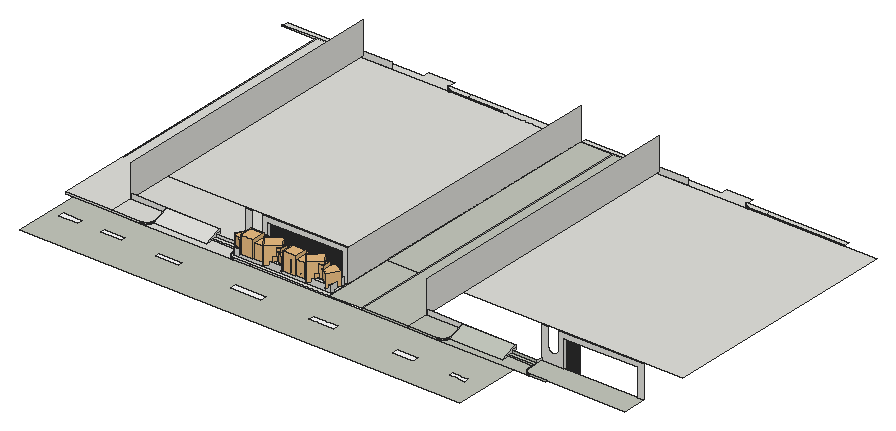
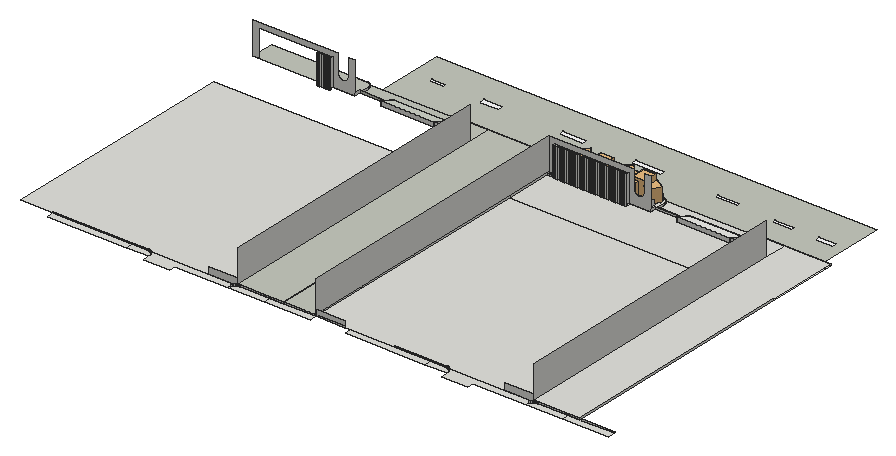
# SketchUp Ruby script. Lengths in inches.
U = 1.inch
M = Sketchup.active_model
def pt(a) = Geom::Point3d.new(a.map { |v| v * U })
def face(e, loops, mat)
  f = e.add_face(loops[0].map { |a| pt(a) })
  loops[1..].each { |l| e.add_face(l.map { |a| pt(a) }).erase! }
  f.material = f.back_material = mat if mat
  f
end
# faces: each face lists its corners as indices into pts; further lists are holes
def faces(e, pts, list, mat = nil) = list.each { |f| face(e, (f[0].is_a?(Array) ? f : [f]).map { |l| l.map { |i| pts[i] } }, mat) }
# xy, xz, yz: faces in a plane at the given z, y or x. An outline is a flat list of corners, or four numbers for a rectangle; further outlines are holes
def ring(l) = l.size == 4 ? [[l[0], l[1]], [l[2], l[1]], [l[2], l[3]], [l[0], l[3]]] : l.each_slice(2).to_a
def flat(e, list, mat, &to3) = list.each { |f| face(e, (f[0].is_a?(Array) ? f : [f]).map { |l| ring(l).map { |u, v| to3.(u, v) } }, mat) }
def xy(e, z, list, mat = nil) = flat(e, list, mat) { |x, y| [x, y, z] }
def xz(e, y, list, mat = nil) = flat(e, list, mat) { |x, z| [x, y, z] }
def yz(e, x, list, mat = nil) = flat(e, list, mat) { |y, z| [x, y, z] }
def lines(e, pts, list) = list.each { |a, b| e.add_line(pt(pts[a]), pt(pts[b])) }
# prism: a flat outline (further loops are holes) pulled along v
def prism(e, loops, v, mat = nil)
  f = face(e, loops, mat); d = Geom::Vector3d.new(v.map { |x| x * U })
  f.pushpull(f.normal.samedirection?(d) ? d.length : -d.length)
end
def box(e, o, s, mat = nil) = prism(e, [[o, [o[0] + s[0], o[1], o[2]], [o[0] + s[0], o[1] + s[1], o[2]], [o[0], o[1] + s[1], o[2]]]], [0, 0, s[2]], mat)
def at(x, y, z, deg = 0) = Geom::Transformation.translation(pt([x, y, z])) * Geom::Transformation.rotation(ORIGIN, Z_AXIS, deg.degrees)
def axes(o, x, y, z) = Geom::Transformation.new([*x, 0, *y, 0, *z, 0, *pt(o).to_a, 1])
def part(name) = M.definitions.add(name)
# library, detail: a bought-in or finely detailed component or shape, given as its bounding box
def library(name, o, s) = part(name).tap { |d| box(d.entities, o, s) }
def detail(e, o, s) = box(e.add_group.entities, o, s)
def put(e, d, t, mat = nil) = e.add_instance(d, t).tap { |i| i.material = mat if mat }
def group(e, t, mat = nil) = e.add_group.tap { |g| g.transformation = t; g.material = mat if mat }.entities
root = M.entities
M.materials.add("Color_000").color = [255, 255, 255]
M.materials.add("Material__1").color = [95, 70, 46]
M.materials.add("[0041_Chocolate]").color = [210, 105, 30]
M.materials.add("[Pavers with Grass Herringbone]").color = [197, 201, 190]
c1 = part("Untitled (5)")
xy(c1.entities,0,[[[158.81,26.5625,306.06,993.3125],[226.57,518.17,239.57,583.92],[225.28,357.51,237.28,411.51],[222.61,182.28,236.36,226.53],[239.71,931.55,251.46,972.3],[233.64,703.93,242.14,755.18],[240.05,835.03,248.8,880.53],[222.04,66.5,231.29,100.5]]])
xy(c1.entities,0,[[222.04,66.5,231.29,100.5],[222.61,182.28,236.36,226.53],[225.28,357.51,237.28,411.51],[226.57,518.17,239.57,583.92],[233.64,703.93,242.14,755.18],
  [240.05,835.03,248.8,880.53],[239.71,931.55,251.46,972.3]],"Color_000")
c2 = library("Areca palm plant",[0,0,0],[49.1,36.6,54.46])
c3 = library("Group\#74",[-84.69,-90.07,-0.36],[176.51,175.13,171.4])
c4 = library("Group20\#1",[-20.81,-17.08,3.79],[39.86,39.43,37.51])
c5 = library("Group38\#2",[14.01,28.44,-23.43],[18.58,18.32,38.89])
c6 = library("Group\#130",[-7.34,-1.2,0],[38.67,35.81,49.04])
c7 = part("Group\#8")
put(c7.entities,c2,axes([-6.2,56.6,6.08],[0.45017,-0.56191,0],[0.66137,0.52986,0],[0,0,0.72]))
put(c7.entities,c2,axes([-6.2,158.41,6.08],[0.45017,-0.56191,0],[0.66137,0.52986,0],[0,0,0.72]))
put(c7.entities,c3,axes([14.93,145.87,6.05],[-0.04961,-0.08593,0],[0.08593,-0.04961,0],[0,0,0.10522]))
put(c7.entities,c3,axes([14.93,193.18,6.05],[-0.04961,-0.08593,0],[0.08593,-0.04961,0],[0,0,0.10522]))
put(c7.entities,c4,axes([18.97,79.98,4.77],[0,0.85,0],[-0.85,0,0],[0,0,0.85]))
put(c7.entities,c3,axes([14.93,173.12,6.05],[-0.04961,-0.08593,0],[0.08593,-0.04961,0],[0,0,0.10522]))
g1 = group(c7.entities,at(0,0,0))
xy(g1,0,[[0,0,6,234.8],[30,0,36,234.8]])
xy(g1,3,[[6,0,30,234.8]])
xy(g1,7,[[6,5,30,229.8]],"Material__1")
xy(g1,15,[[[0,0,36,234.8],[6,5,30,229.8]]])
xz(g1,0,[[0,0,6,0,6,3,30,3,30,0,36,0,36,15,0,15]])
xz(g1,5,[[6,7,30,15]])
xz(g1,229.8,[[6,7,30,15]])
xz(g1,234.8,[[0,0,0,15,36,15,36,0,30,0,30,3,6,3,6,0]])
yz(g1,0,[[0,0,234.8,15]])
yz(g1,6,[[0,0,234.8,3],[5,7,229.8,15]])
yz(g1,30,[[0,0,234.8,3],[5,7,229.8,15]])
yz(g1,36,[[0,0,234.8,15]])
put(c7.entities,c3,axes([17.19,223.04,6.07],[-0.08133,-0.14087,0],[0.14087,-0.08133,0],[0,0,0.1725]))
put(c7.entities,c5,axes([-4.1,-1.15,28.17],[0.8848,0,0],[0,0.94674,0],[0,0,0.85826]))
put(c7.entities,c3,axes([17.19,15.79,6.07],[-0.08133,-0.14087,0],[0.14087,-0.08133,0],[0,0,0.1725]))
put(c7.entities,c3,axes([14.93,91.37,6.05],[-0.04961,-0.08593,0],[0.08593,-0.04961,0],[0,0,0.10522]))
put(c7.entities,c4,axes([18.97,181.79,4.77],[0,0.85,0],[-0.85,0,0],[0,0,0.85]))
put(c7.entities,c3,axes([14.93,44.05,6.05],[-0.04961,-0.08593,0],[0.08593,-0.04961,0],[0,0,0.10522]))
put(c7.entities,c6,axes([24.9375,191.72,8],[0,0.79,0],[-0.79,0,0],[0,0,0.79]))
put(c7.entities,c3,axes([17.19,121.23,6.07],[-0.08133,-0.14087,0],[0.14087,-0.08133,0],[0,0,0.1725]))
put(c7.entities,c5,axes([-4.1,100.66,28.17],[0.8848,0,0],[0,0.94674,0],[0,0,0.85826]))
put(c7.entities,c6,axes([24.9375,89.91,8],[0,0.79,0],[-0.79,0,0],[0,0,0.79]))
put(c7.entities,c3,axes([14.93,71.3,6.05],[-0.04961,-0.08593,0],[0.08593,-0.04961,0],[0,0,0.10522]))
xy(root,-8,[[484.21,147.25,585.4,162.52],[585.4,147.25,649.69,147.25,651.69,147.38,653.64,147.77,655.53,148.41,657.33,149.3,658.99,150.4,660.49,151.72,661.8,153.22,662.91,154.88,663.8,156.67,664.4375,158.57,664.83,160.52,664.96,162.52,585.4,162.52],[649.69,147.25,854.5,147.25,852.53,147.38,850.6,147.76,848.73,148.4,846.96,149.27,845.32,150.37,843.84,151.67,842.53,153.15,841.4375,154.79,840.57,156.56,839.93,158.43,839.55,160.36,839.42,162.33,839.42,178.0625,782.4,178.0625,782.4,162.52,664.96,162.52,664.83,160.52,664.4375,158.57,663.8,156.67,662.91,154.88,661.8,153.22,660.49,151.72,658.99,150.4,657.33,149.3,655.53,148.41,653.64,147.77,651.69,147.38],[854.5,147.25,888.5,147.25,888.5,162.33,839.42,162.33,839.55,160.36,839.93,158.43,840.57,156.56,841.4375,154.79,842.53,153.15,843.84,151.67,845.32,150.37,846.96,149.27,848.73,148.4,850.6,147.76,852.53,147.38],[888.5,147.25,1063.02,162.33],
  [1134.71,147.25,1235.9,162.52],[1235.9,147.25,1300.19,147.25,1302.19,147.38,1304.14,147.77,1306.03,148.41,1307.83,149.3,1309.49,150.4,1310.99,151.72,1312.3,153.22,1313.41,154.88,1314.3,156.67,1314.9375,158.57,1315.33,160.52,1315.46,162.52,1235.9,162.52],[1505,147.25,1539,147.25,1539,162.33,1489.92,162.33,1490.05,160.36,1490.43,158.43,1491.07,156.56,1491.9375,154.79,1493.03,153.15,1494.34,151.67,1495.82,150.37,1497.46,149.27,1499.23,148.4,1501.1,147.76,1503.03,147.38],[839.42,162.33,888.5,162.33,888.5,203.875,890.125,203.875,890.125,204.875,890.875,204.875,890.875,203.875,894.125,203.875,894.125,204.875,894.875,204.875,894.875,203.875,898.125,203.875,898.125,204.875,898.875,204.875,898.875,203.875,902.125,203.875,902.125,204.875,902.875,204.875,902.875,203.875,906.125,203.875,906.125,204.875,906.875,204.875,906.875,203.875,910.125,203.875,910.125,204.875,910.875,204.875,910.875,203.875,914.125,203.875,914.125,204.875,914.875,204.875,914.875,203.875,918.125,203.875,918.125,204.875,918.875,204.875,918.875,203.875,922.125,203.875,922.125,204.875,922.875,204.875,922.875,203.875,926.125,203.875,926.125,204.875,926.875,204.875,926.875,203.875,930.125,203.875,930.125,204.875,930.875,204.875,930.875,203.875,934.125,203.875,934.125,204.875,934.875,204.875,934.875,203.875,938.125,203.875,938.125,204.875,938.875,204.875,938.875,203.875,942.125,203.875,942.125,204.875,942.875,204.875,942.875,203.875,946.125,203.875,946.125,204.875,946.875,204.875,946.875,203.875,950.125,203.875,950.125,204.875,950.875,204.875,950.875,203.875,954.125,203.875,954.125,204.875,954.875,204.875,954.875,203.875,958.125,203.875,958.125,204.875,958.875,204.875,958.875,203.875,962.125,203.875,962.125,204.875,962.875,204.875,962.875,203.875,966.125,203.875,966.125,204.875,966.875,204.875,966.875,203.875,970.125,203.875,970.125,204.875,970.875,204.875,970.875,203.875,974.125,203.875,974.125,204.875,974.875,204.875,974.875,203.875,978.125,203.875,978.125,204.875,978.875,204.875,978.875,203.875,982.125,203.875,982.125,204.875,982.875,204.875,982.875,203.875,986.125,203.875,986.125,204.875,986.875,204.875,986.875,203.875,990.125,203.875,990.125,204.875,990.875,204.875,990.875,203.875,994.125,203.875,994.125,204.875,994.875,204.875,994.875,203.875,998.125,203.875,998.125,204.875,998.875,204.875,998.875,203.875,1002.125,203.875,1002.125,204.875,1002.875,204.875,1002.875,203.875,1006.125,203.875,1006.125,204.875,1006.875,204.875,1006.875,203.875,1010.125,203.875,1010.125,204.875,1010.875,204.875,1010.875,203.875,1014.125,203.875,1014.125,204.875,1014.875,204.875,1014.875,203.875,1018.125,203.875,1018.125,204.875,1018.875,204.875,1018.875,203.875,1022.125,203.875,1022.125,204.875,1022.875,204.875,1022.875,203.875,1026.125,203.875,1026.125,204.875,1026.875,204.875,1026.875,203.875,1030.125,203.875,1030.125,204.875,1030.875,204.875,1030.875,203.875,1034.125,203.875,1034.125,204.875,1034.875,204.875,1034.875,203.875,1038.125,203.875,1038.125,204.875,1038.875,204.875,1038.875,203.875,1042.125,203.875,1042.125,204.875,1042.875,204.875,1042.875,203.875,1046.125,203.875,1046.125,204.875,1046.875,204.875,1046.875,203.875,1063.02,203.875,1063.02,305.58,484.21,305.58,484.21,162.52,782.4,162.52,782.4,178.0625,839.42,178.0625],[888.5,162.33,888.5,203.875,1050.125,203.875,1050.125,198.625,1063.02,198.625,1063.02,162.33],
  [1050.125,198.625,1063.02,203.875],[484.21,305.58,1063.02,838.14],[1134.71,305.58,1713.52,838.14],[407.52,838.14,508.71,853.41],[508.71,838.14,573,838.14,575,838.27,576.96,838.66,578.85,839.31,580.64,840.19,582.3,841.3,583.8,842.62,585.12,844.12,586.23,845.78,587.11,847.57,587.75,849.46,588.14,851.42,588.27,853.41,508.71,853.41],
  [573,838.14,777.8125,838.14,775.84,838.27,773.91,838.66,772.04,839.29,770.27,840.16,768.63,841.26,767.15,842.5625,765.85,844.04,764.75,845.68,763.88,847.45,763.24,849.32,762.86,851.26,762.73,853.22,762.73,868.96,705.71,868.96,705.71,853.41,588.27,853.41,588.14,851.42,587.75,849.46,587.11,847.57,586.23,845.78,585.12,844.12,583.8,842.62,582.3,841.3,580.64,840.19,578.85,839.31,576.96,838.66,575,838.27],[777.8125,838.14,811.8125,838.14,811.8125,853.22,762.73,853.22,762.86,851.26,763.24,849.32,763.88,847.45,764.75,845.68,765.85,844.04,767.15,842.5625,768.63,841.26,770.27,840.16,772.04,839.29,773.91,838.66,775.84,838.27],[811.8125,838.14,986.33,853.22],[1063.02,838.14,1164.21,853.41],[1164.21,838.14,1228.5,838.14,1230.5,838.27,1232.46,838.66,1234.35,839.31,1236.14,840.19,1237.8,841.3,1239.3,842.62,1240.62,844.12,1241.73,845.78,1242.61,847.57,1243.25,849.46,1243.64,851.42,1243.77,853.41,1164.21,853.41],
  [1228.5,838.14,1433.3125,838.14,1431.34,838.27,1429.41,838.66,1427.54,839.29,1425.77,840.16,1424.13,841.26,1422.65,842.5625,1421.35,844.04,1420.25,845.68,1419.38,847.45,1418.74,849.32,1418.36,851.26,1418.23,853.22,1418.23,868.96,1361.21,868.96,1361.21,853.41,1243.77,853.41,1243.64,851.42,1243.25,849.46,1242.61,847.57,1241.73,845.78,1240.62,844.12,1239.3,842.62,1237.8,841.3,1236.14,840.19,1234.35,839.31,1232.46,838.66,1230.5,838.27],[1433.3125,838.14,1467.3125,838.14,1467.3125,853.22,1418.23,853.22,1418.36,851.26,1418.74,849.32,1419.38,847.45,1420.25,845.68,1421.35,844.04,1422.65,842.5625,1424.13,841.26,1425.77,840.16,1427.54,839.29,1429.41,838.66,1431.34,838.27],[1467.3125,838.14,1641.83,853.22]])
xy(root,-8,[[1300.19,147.25,1505,147.25,1503.03,147.38,1501.1,147.76,1499.23,148.4,1497.46,149.27,1495.82,150.37,1494.34,151.67,1493.03,153.15,1491.9375,154.79,1491.07,156.56,1490.43,158.43,1490.05,160.36,1489.92,162.33,1489.92,178.0625,1432.9,178.0625,1432.9,162.52,1315.46,162.52,1315.33,160.52,1314.9375,158.57,1314.3,156.67,1313.41,154.88,1312.3,153.22,1310.99,151.72,1309.49,150.4,1307.83,149.3,1306.03,148.41,1304.14,147.77,1302.19,147.38]],"[Pavers with Grass Herringbone]")
xy(root,-4.67,[[484.21,147.25,585.4,838.14],[585.4,147.25,649.69,147.25,651.69,147.38,653.64,147.77,655.53,148.41,657.33,149.3,658.99,150.4,660.49,151.72,661.8,153.22,662.91,154.88,663.8,156.67,664.4375,158.57,664.83,160.52,664.96,162.52,664.96,198.625,585.4,198.625],[854.5,147.25,1063.02,147.25,1063.02,198.625,839.42,198.625,839.42,162.33,839.55,160.36,839.93,158.43,840.57,156.56,841.4375,154.79,842.53,153.15,843.84,151.67,845.32,150.37,846.96,149.27,848.73,148.4,850.6,147.76,852.53,147.38],[782.4,178.0625,839.42,185.9375],[888.5,198.625,1063.02,203.875]])
xy(root,-4.67,[[1063.02,147.25,1134.71,305.58],[1134.71,147.25,1235.9,838.14],[1235.9,147.25,1300.19,147.25,1302.19,147.38,1304.14,147.77,1306.03,148.41,1307.83,149.3,1309.49,150.4,1310.99,151.72,1312.3,153.22,1313.41,154.88,1314.3,156.67,1314.9375,158.57,1315.33,160.52,1315.46,162.52,1315.46,198.625,1235.9,198.625],[1505,147.25,1713.52,147.25,1713.52,198.625,1489.92,198.625,1489.92,162.33,1490.05,160.36,1490.43,158.43,1491.07,156.56,1491.9375,154.79,1493.03,153.15,1494.34,151.67,1495.82,150.37,1497.46,149.27,1499.23,148.4,1501.1,147.76,1503.03,147.38],[1432.9,178.0625,1489.92,185.9375],
  [1063.02,305.58,1134.71,838.14]],"[Pavers with Grass Herringbone]")
xz(root,147.25,[[484.21,-8,585.4,-4.67],[585.4,-8,649.69,-4.67],[854.5,-8,888.5,-4.67],[888.5,-8,1063.02,-4.67]])
xz(root,147.25,[[1134.71,-8,1235.9,-4.67],[1235.9,-8,1300.19,-4.67],[1505,-8,1539,-4.67]],"[Pavers with Grass Herringbone]")
xz(root,178.0625,[[782.4,-8,839.42,-4.67]])
xz(root,178.0625,[[1432.9,-8,1489.92,-4.67]],"[Pavers with Grass Herringbone]")
xz(root,185.9375,[[782.4,-4.67,839.42,0.73]])
xz(root,185.9375,[[1432.9,-4.67,1489.92,0.73]],"[Pavers with Grass Herringbone]")
xz(root,198.625,[[1050.125,-8,1063.02,-4.67],[585.4,-4.67,664.96,6.125],[664.96,-4.67,782.4,6.125],[839.42,-4.67,888.5,-4.67,888.5,55.1875,1050.125,55.1875,1050.125,-4.67,1063.02,-4.67,1063.02,66.125,877.1,66.125,877.1,26.79,876.21,24.11,874.74,21.71,872.77,19.69,870.4,18.17,867.74,17.23,864.94,16.91,862.14,17.23,859.49,18.17,857.11,19.69,855.14,21.71,853.67,24.11,852.79,26.79,852.79,66.125,839.66,66.125,839.66,6.125,839.42,6.125],[1235.9,-4.67,1315.46,6.125],
  [1315.46,-4.67,1432.9,6.125],[1489.92,-4.67,1539,-4.67,1539,55.1875,1700.625,55.1875,1700.625,-4.67,1713.52,-4.67,1713.52,66.125,1527.6,66.125,1527.6,26.79,1526.71,24.11,1525.24,21.71,1523.27,19.69,1520.9,18.17,1518.24,17.23,1515.44,16.91,1512.64,17.23,1509.99,18.17,1507.61,19.69,1505.64,21.71,1504.17,24.11,1503.29,26.79,1503.29,66.125,1490.16,66.125,1490.16,6.125,1489.92,6.125]])
xz(root,203.875,[[888.5,-8,890.125,-4.67],[890.125,-8,890.875,-4.67],[890.875,-8,894.125,-4.67],[894.125,-8,894.875,-4.67],[894.875,-8,898.125,-4.67],
  [898.125,-8,898.875,-4.67],[898.875,-8,902.125,-4.67],[902.125,-8,902.875,-4.67],[902.875,-8,906.125,-4.67],[906.125,-8,906.875,-4.67],
  [906.875,-8,910.125,-4.67],[910.125,-8,910.875,-4.67],[910.875,-8,914.125,-4.67],[914.125,-8,914.875,-4.67],[914.875,-8,918.125,-4.67],
  [918.125,-8,918.875,-4.67],[918.875,-8,922.125,-4.67],[922.125,-8,922.875,-4.67],[922.875,-8,926.125,-4.67],[926.125,-8,926.875,-4.67],
  [926.875,-8,930.125,-4.67],[930.125,-8,930.875,-4.67],[930.875,-8,934.125,-4.67],[934.125,-8,934.875,-4.67],[934.875,-8,938.125,-4.67],
  [938.125,-8,938.875,-4.67],[938.875,-8,942.125,-4.67],[942.125,-8,942.875,-4.67],[942.875,-8,946.125,-4.67],[946.125,-8,946.875,-4.67],
  [946.875,-8,950.125,-4.67],[950.125,-8,950.875,-4.67],[950.875,-8,954.125,-4.67],[954.125,-8,954.875,-4.67],[954.875,-8,958.125,-4.67],
  [958.125,-8,958.875,-4.67],[958.875,-8,962.125,-4.67],[962.125,-8,962.875,-4.67],[962.875,-8,966.125,-4.67],[966.125,-8,966.875,-4.67],
  [966.875,-8,970.125,-4.67],[970.125,-8,970.875,-4.67],[970.875,-8,974.125,-4.67],[974.125,-8,974.875,-4.67],[974.875,-8,978.125,-4.67],
  [978.125,-8,978.875,-4.67],[978.875,-8,982.125,-4.67],[982.125,-8,982.875,-4.67],[982.875,-8,986.125,-4.67],[986.125,-8,986.875,-4.67],
  [986.875,-8,990.125,-4.67],[990.125,-8,990.875,-4.67],[990.875,-8,994.125,-4.67],[994.125,-8,994.875,-4.67],[994.875,-8,998.125,-4.67],
  [998.125,-8,998.875,-4.67],[998.875,-8,1002.125,-4.67],[1002.125,-8,1002.875,-4.67],[1002.875,-8,1006.125,-4.67],[1006.125,-8,1006.875,-4.67],
  [1006.875,-8,1010.125,-4.67],[1010.125,-8,1010.875,-4.67],[1010.875,-8,1014.125,-4.67],[1014.125,-8,1014.875,-4.67],[1014.875,-8,1018.125,-4.67],
  [1018.125,-8,1018.875,-4.67],[1018.875,-8,1022.125,-4.67],[1022.125,-8,1022.875,-4.67],[1022.875,-8,1026.125,-4.67],[1026.125,-8,1026.875,-4.67],
  [1026.875,-8,1030.125,-4.67],[1030.125,-8,1030.875,-4.67],[1030.875,-8,1034.125,-4.67],[1034.125,-8,1034.875,-4.67],[1034.875,-8,1038.125,-4.67],
  [1038.125,-8,1038.875,-4.67],[1038.875,-8,1042.125,-4.67],[1042.125,-8,1042.875,-4.67],[1042.875,-8,1046.125,-4.67],[1046.125,-8,1046.875,-4.67],
  [1046.875,-8,1050.125,-4.67],[1050.125,-8,1063.02,-4.67],[1539,-8,1540.625,-4.67],[1540.625,-8,1541.375,-4.67],[1541.375,-8,1544.625,-4.67],
  [1544.625,-8,1545.375,-4.67],[1545.375,-8,1548.625,-4.67],[1548.625,-8,1549.375,-4.67],[1549.375,-8,1552.625,-4.67],[1552.625,-8,1553.375,-4.67],
  [1553.375,-8,1556.625,-4.67],[1556.625,-8,1557.375,-4.67],[1557.375,-8,1560.625,-4.67],[1560.625,-8,1561.375,-4.67],[1561.375,-8,1564.625,-4.67],
  [1564.625,-8,1565.375,-4.67],[1565.375,-8,1568.625,-4.67],[1568.625,-8,1569.375,-4.67]])
xz(root,203.875,[[888.5,-4.67,890.125,55.1875],[890.875,-4.67,894.125,55.1875],[894.875,-4.67,898.125,55.1875],[898.875,-4.67,902.125,55.1875],[902.875,-4.67,906.125,55.1875],
  [906.875,-4.67,910.125,55.1875],[910.875,-4.67,914.125,55.1875],[914.875,-4.67,918.125,55.1875],[918.875,-4.67,922.125,55.1875],[922.875,-4.67,926.125,55.1875],
  [926.875,-4.67,930.125,55.1875],[930.875,-4.67,934.125,55.1875],[934.875,-4.67,938.125,55.1875],[938.875,-4.67,942.125,55.1875],[942.875,-4.67,946.125,55.1875],
  [946.875,-4.67,950.125,55.1875],[950.875,-4.67,954.125,55.1875],[954.875,-4.67,958.125,55.1875],[958.875,-4.67,962.125,55.1875],[962.875,-4.67,966.125,55.1875],
  [966.875,-4.67,970.125,55.1875],[970.875,-4.67,974.125,55.1875],[974.875,-4.67,978.125,55.1875],[978.875,-4.67,982.125,55.1875],[982.875,-4.67,986.125,55.1875],
  [986.875,-4.67,990.125,55.1875],[990.875,-4.67,994.125,55.1875],[994.875,-4.67,998.125,55.1875],[998.875,-4.67,1002.125,55.1875],[1002.875,-4.67,1006.125,55.1875],
  [1006.875,-4.67,1010.125,55.1875],[1010.875,-4.67,1014.125,55.1875],[1014.875,-4.67,1018.125,55.1875],[1018.875,-4.67,1022.125,55.1875],[1022.875,-4.67,1026.125,55.1875],
  [1026.875,-4.67,1030.125,55.1875],[1030.875,-4.67,1034.125,55.1875],[1034.875,-4.67,1038.125,55.1875],[1038.875,-4.67,1042.125,55.1875],[1042.875,-4.67,1046.125,55.1875],
  [1046.875,-4.67,1050.125,55.1875],[1539,-4.67,1540.625,55.1875],[1541.375,-4.67,1544.625,55.1875],[1545.375,-4.67,1548.625,55.1875],[1549.375,-4.67,1552.625,55.1875],
  [1553.375,-4.67,1556.625,55.1875],[1557.375,-4.67,1560.625,55.1875],[1561.375,-4.67,1564.625,55.1875],[1565.375,-4.67,1568.625,55.1875]],"[0041_Chocolate]")
xz(root,204.875,[[890.125,-8,890.875,55.1875],[894.125,-8,894.875,55.1875],[898.125,-8,898.875,55.1875],[902.125,-8,902.875,55.1875],[906.125,-8,906.875,55.1875],
  [910.125,-8,910.875,55.1875],[914.125,-8,914.875,55.1875],[918.125,-8,918.875,55.1875],[922.125,-8,922.875,55.1875],[926.125,-8,926.875,55.1875],
  [930.125,-8,930.875,55.1875],[934.125,-8,934.875,55.1875],[938.125,-8,938.875,55.1875],[942.125,-8,942.875,55.1875],[946.125,-8,946.875,55.1875],
  [950.125,-8,950.875,55.1875],[954.125,-8,954.875,55.1875],[958.125,-8,958.875,55.1875],[962.125,-8,962.875,55.1875],[966.125,-8,966.875,55.1875],
  [970.125,-8,970.875,55.1875],[974.125,-8,974.875,55.1875],[978.125,-8,978.875,55.1875],[982.125,-8,982.875,55.1875],[986.125,-8,986.875,55.1875],
  [990.125,-8,990.875,55.1875],[994.125,-8,994.875,55.1875],[998.125,-8,998.875,55.1875],[1002.125,-8,1002.875,55.1875],[1006.125,-8,1006.875,55.1875],
  [1010.125,-8,1010.875,55.1875],[1014.125,-8,1014.875,55.1875],[1018.125,-8,1018.875,55.1875],[1022.125,-8,1022.875,55.1875],[1026.125,-8,1026.875,55.1875],
  [1030.125,-8,1030.875,55.1875],[1034.125,-8,1034.875,55.1875],[1038.125,-8,1038.875,55.1875],[1042.125,-8,1042.875,55.1875],[1046.125,-8,1046.875,55.1875],
  [1540.625,-8,1541.375,55.1875],[1544.625,-8,1545.375,55.1875],[1548.625,-8,1549.375,55.1875],[1552.625,-8,1553.375,55.1875],[1556.625,-8,1557.375,55.1875],
  [1560.625,-8,1561.375,55.1875],[1564.625,-8,1565.375,55.1875],[1568.625,-8,1569.375,55.1875]])
xz(root,838.14,[[407.52,-8,479.21,-4.67],[484.21,-8,508.71,-4.67],[508.71,-8,539.77,-4.67],[539.77,-8,573,-4.67],[573,-8,573,-4.67,585.4,-4.67,585.4,6.125,648.9,6.125,648.9,-8],
  [777.8125,-8,811.8125,-4.67],[811.8125,-8,890.4,-4.67],[1058.02,-8,1058.02,-4.67,999.52,-4.67,999.52,6.125,1063.02,6.125,1063.02,-8],[999.52,-8,1058.02,-4.67],[1063.02,-8,1134.71,-4.67],
  [1134.71,-8,1164.21,-4.67],[1164.21,-8,1228.5,-4.67],[1228.5,-8,1228.5,-4.67,1235.9,-4.67,1235.9,6.125,1299.4,6.125,1299.4,-8],[1433.3125,-8,1467.3125,-4.67],[1467.3125,-8,1641.83,-4.67]])
yz(root,484.21,[[305.58,-8,838.14,-4.67]])
yz(root,585.4,[[198.625,-4.67,838.14,66.125]])
yz(root,664.96,[[162.52,-8,171.04,-4.67,162.52,-4.67],[171.04,-4.67,198.625,6.125,198.625,-4.67]])
yz(root,782.4,[[162.52,-8,178.0625,-8,178.0625,-4.67,171.04,-4.67],[171.04,-4.67,185.9375,-4.67,185.9375,0.73,198.625,0.73,198.625,6.125],[185.9375,-4.67,198.625,0.73]])
yz(root,839.42,[[162.33,-8,178.0625,-4.67],[185.9375,-4.67,198.625,0.73]])
yz(root,888.5,[[198.625,-4.67,203.875,55.1875]])
yz(root,890.125,[[203.875,-8,204.875,55.1875]])
yz(root,890.875,[[203.875,-8,204.875,55.1875]])
yz(root,894.125,[[203.875,-8,204.875,55.1875]])
yz(root,894.875,[[203.875,-8,204.875,55.1875]])
yz(root,898.125,[[203.875,-8,204.875,55.1875]])
yz(root,898.875,[[203.875,-8,204.875,55.1875]])
yz(root,902.125,[[203.875,-8,204.875,55.1875]])
yz(root,902.875,[[203.875,-8,204.875,55.1875]])
yz(root,906.125,[[203.875,-8,204.875,55.1875]])
yz(root,906.875,[[203.875,-8,204.875,55.1875]])
yz(root,910.125,[[203.875,-8,204.875,55.1875]])
yz(root,910.875,[[203.875,-8,204.875,55.1875]])
yz(root,914.125,[[203.875,-8,204.875,55.1875]])
yz(root,914.875,[[203.875,-8,204.875,55.1875]])
yz(root,918.125,[[203.875,-8,204.875,55.1875]])
yz(root,918.875,[[203.875,-8,204.875,55.1875]])
yz(root,922.125,[[203.875,-8,204.875,55.1875]])
yz(root,922.875,[[203.875,-8,204.875,55.1875]])
yz(root,926.125,[[203.875,-8,204.875,55.1875]])
yz(root,926.875,[[203.875,-8,204.875,55.1875]])
yz(root,930.125,[[203.875,-8,204.875,55.1875]])
yz(root,930.875,[[203.875,-8,204.875,55.1875]])
yz(root,934.125,[[203.875,-8,204.875,55.1875]])
yz(root,934.875,[[203.875,-8,204.875,55.1875]])
yz(root,938.125,[[203.875,-8,204.875,55.1875]])
yz(root,938.875,[[203.875,-8,204.875,55.1875]])
yz(root,942.125,[[203.875,-8,204.875,55.1875]])
yz(root,942.875,[[203.875,-8,204.875,55.1875]])
yz(root,946.125,[[203.875,-8,204.875,55.1875]])
yz(root,946.875,[[203.875,-8,204.875,55.1875]])
yz(root,950.125,[[203.875,-8,204.875,55.1875]])
yz(root,950.875,[[203.875,-8,204.875,55.1875]])
yz(root,954.125,[[203.875,-8,204.875,55.1875]])
yz(root,954.875,[[203.875,-8,204.875,55.1875]])
yz(root,958.125,[[203.875,-8,204.875,55.1875]])
yz(root,958.875,[[203.875,-8,204.875,55.1875]])
yz(root,962.125,[[203.875,-8,204.875,55.1875]])
yz(root,962.875,[[203.875,-8,204.875,55.1875]])
yz(root,966.125,[[203.875,-8,204.875,55.1875]])
yz(root,966.875,[[203.875,-8,204.875,55.1875]])
yz(root,970.125,[[203.875,-8,204.875,55.1875]])
yz(root,970.875,[[203.875,-8,204.875,55.1875]])
yz(root,974.125,[[203.875,-8,204.875,55.1875]])
yz(root,974.875,[[203.875,-8,204.875,55.1875]])
yz(root,978.125,[[203.875,-8,204.875,55.1875]])
yz(root,978.875,[[203.875,-8,204.875,55.1875]])
yz(root,982.125,[[203.875,-8,204.875,55.1875]])
yz(root,982.875,[[203.875,-8,204.875,55.1875]])
yz(root,986.125,[[203.875,-8,204.875,55.1875]])
yz(root,986.875,[[203.875,-8,204.875,55.1875]])
yz(root,990.125,[[203.875,-8,204.875,55.1875]])
yz(root,990.875,[[203.875,-8,204.875,55.1875]])
yz(root,994.125,[[203.875,-8,204.875,55.1875]])
yz(root,994.875,[[203.875,-8,204.875,55.1875]])
yz(root,998.125,[[203.875,-8,204.875,55.1875]])
yz(root,998.875,[[203.875,-8,204.875,55.1875]])
yz(root,1002.125,[[203.875,-8,204.875,55.1875]])
yz(root,1002.875,[[203.875,-8,204.875,55.1875]])
yz(root,1006.125,[[203.875,-8,204.875,55.1875]])
yz(root,1006.875,[[203.875,-8,204.875,55.1875]])
yz(root,1010.125,[[203.875,-8,204.875,55.1875]])
yz(root,1010.875,[[203.875,-8,204.875,55.1875]])
yz(root,1014.125,[[203.875,-8,204.875,55.1875]])
yz(root,1014.875,[[203.875,-8,204.875,55.1875]])
yz(root,1018.125,[[203.875,-8,204.875,55.1875]])
yz(root,1018.875,[[203.875,-8,204.875,55.1875]])
yz(root,1022.125,[[203.875,-8,204.875,55.1875]])
yz(root,1022.875,[[203.875,-8,204.875,55.1875]])
yz(root,1026.125,[[203.875,-8,204.875,55.1875]])
yz(root,1026.875,[[203.875,-8,204.875,55.1875]])
yz(root,1030.125,[[203.875,-8,204.875,55.1875]])
yz(root,1030.875,[[203.875,-8,204.875,55.1875]])
yz(root,1034.125,[[203.875,-8,204.875,55.1875]])
yz(root,1034.875,[[203.875,-8,204.875,55.1875]])
yz(root,1038.125,[[203.875,-8,204.875,55.1875]])
yz(root,1038.875,[[203.875,-8,204.875,55.1875]])
yz(root,1042.125,[[203.875,-8,204.875,55.1875]])
yz(root,1042.875,[[203.875,-8,204.875,55.1875]])
yz(root,1046.125,[[203.875,-8,204.875,55.1875]])
yz(root,1046.875,[[203.875,-8,204.875,55.1875]])
yz(root,1050.125,[[198.625,-8,203.875,55.1875]])
yz(root,1063.02,[[147.25,-8,198.625,-4.67],[198.625,-8,203.875,-4.67],[203.875,-8,305.58,-4.67],[305.58,-8,838.14,-4.67],[198.625,-4.67,838.14,66.125]])
yz(root,1134.71,[[147.25,-8,305.58,-4.67],[305.58,-8,838.14,-4.67]])
yz(root,1235.9,[[198.625,-4.67,838.14,66.125]])
yz(root,1315.46,[[162.52,-8,171.04,-4.67,162.52,-4.67],[171.04,-4.67,198.625,6.125,198.625,-4.67]])
yz(root,1432.9,[[162.52,-8,178.0625,-8,178.0625,-4.67,171.04,-4.67],[171.04,-4.67,185.9375,-4.67,185.9375,0.73,198.625,0.73,198.625,6.125],[185.9375,-4.67,198.625,0.73]])
yz(root,1489.92,[[162.33,-8,178.0625,-4.67],[185.9375,-4.67,198.625,0.73]])
yz(root,1539,[[198.625,-4.67,203.875,55.1875]])
yz(root,1540.625,[[203.875,-8,204.875,55.1875]])
yz(root,1541.375,[[203.875,-8,204.875,55.1875]])
yz(root,1544.625,[[203.875,-8,204.875,55.1875]])
yz(root,1545.375,[[203.875,-8,204.875,55.1875]])
yz(root,1548.625,[[203.875,-8,204.875,55.1875]])
yz(root,1549.375,[[203.875,-8,204.875,55.1875]])
yz(root,1552.625,[[203.875,-8,204.875,55.1875]])
yz(root,1553.375,[[203.875,-8,204.875,55.1875]])
yz(root,1556.625,[[203.875,-8,204.875,55.1875]])
yz(root,1557.375,[[203.875,-8,204.875,55.1875]])
yz(root,1560.625,[[203.875,-8,204.875,55.1875]])
yz(root,1561.375,[[203.875,-8,204.875,55.1875]])
yz(root,1564.625,[[203.875,-8,204.875,55.1875]])
yz(root,1565.375,[[203.875,-8,204.875,55.1875]])
yz(root,1568.625,[[203.875,-8,204.875,55.1875]])
yz(root,1569.375,[[203.875,-8,204.875,55.1875]])
p = [[651.69,147.38,-4.67],[649.69,147.25,-4.67],[649.69,147.25,-8],[651.69,147.38,-8],[854.5,147.25,-4.67],[852.53,147.38,-4.67],
  [852.53,147.38,-8],[854.5,147.25,-8],[1302.19,147.38,-4.67],[1300.19,147.25,-4.67],[1300.19,147.25,-8],[1302.19,147.38,-8],
  [1505,147.25,-4.67],[1503.03,147.38,-4.67],[1503.03,147.38,-8],[1505,147.25,-8],[653.64,147.77,-4.67],[653.64,147.77,-8],
  [850.6,147.76,-4.67],[850.6,147.76,-8],[1304.14,147.77,-4.67],[1304.14,147.77,-8],[1501.1,147.76,-4.67],[1501.1,147.76,-8],
  [655.53,148.41,-4.67],[655.53,148.41,-8],[848.73,148.4,-4.67],[848.73,148.4,-8],[1306.03,148.41,-4.67],[1306.03,148.41,-8],
  [1499.23,148.4,-4.67],[1499.23,148.4,-8],[657.33,149.3,-4.67],[657.33,149.3,-8],[846.96,149.27,-4.67],[846.96,149.27,-8],
  [1307.83,149.3,-4.67],[1307.83,149.3,-8],[1497.46,149.27,-4.67],[1497.46,149.27,-8],[658.99,150.4,-4.67],[658.99,150.4,-8],
  [845.32,150.37,-4.67],[845.32,150.37,-8],[1309.49,150.4,-4.67],[1309.49,150.4,-8],[1495.82,150.37,-4.67],[1495.82,150.37,-8],
  [660.49,151.72,-4.67],[660.49,151.72,-8],[843.84,151.67,-4.67],[843.84,151.67,-8],[1310.99,151.72,-4.67],[1310.99,151.72,-8],
  [1494.34,151.67,-4.67],[1494.34,151.67,-8],[661.8,153.22,-4.67],[661.8,153.22,-8],[842.53,153.15,-4.67],[842.53,153.15,-8],
  [1312.3,153.22,-4.67],[1312.3,153.22,-8],[1493.03,153.15,-4.67],[1493.03,153.15,-8],[662.91,154.88,-4.67],[662.91,154.88,-8],
  [841.4375,154.79,-4.67],[841.4375,154.79,-8],[1313.41,154.88,-4.67],[1313.41,154.88,-8],[1491.9375,154.79,-4.67],[1491.9375,154.79,-8],
  [840.57,156.56,-4.67],[840.57,156.56,-8],[1491.07,156.56,-4.67],[1491.07,156.56,-8],[663.8,156.67,-4.67],[663.8,156.67,-8],
  [1314.3,156.67,-4.67],[1314.3,156.67,-8],[839.93,158.43,-4.67],[839.93,158.43,-8],[1490.43,158.43,-4.67],[1490.43,158.43,-8],
  [664.4375,158.57,-4.67],[664.4375,158.57,-8],[1314.9375,158.57,-4.67],[1314.9375,158.57,-8],[839.55,160.36,-4.67],[839.55,160.36,-8],
  [1490.05,160.36,-4.67],[1490.05,160.36,-8],[664.83,160.52,-4.67],[664.83,160.52,-8],[1315.33,160.52,-4.67],[1315.33,160.52,-8],
  [839.42,162.33,-4.67],[839.42,162.33,-8],[1489.92,162.33,-4.67],[1489.92,162.33,-8],[664.96,162.52,-4.67],[664.96,162.52,-8],
  [1315.46,162.52,-4.67],[1315.46,162.52,-8],[782.4,162.52,-8],[782.4,171.04,-4.67],[782.4,198.625,6.125],[664.96,198.625,6.125],
  [664.96,171.04,-4.67],[1432.9,162.52,-8],[1432.9,171.04,-4.67],[1432.9,198.625,6.125],[1315.46,198.625,6.125],[1315.46,171.04,-4.67],
  [575,838.27,-4.67],[573,838.14,-4.67],[573,838.14,-8],[575,838.27,-8],[777.8125,838.14,-4.67],[775.84,838.27,-4.67],
  [775.84,838.27,-8],[777.8125,838.14,-8],[1230.5,838.27,-4.67],[1228.5,838.14,-4.67],[1228.5,838.14,-8],[1230.5,838.27,-8],
  [1433.3125,838.14,-4.67],[1431.34,838.27,-4.67],[1431.34,838.27,-8],[1433.3125,838.14,-8],[576.96,838.66,-4.67],[576.96,838.66,-8],
  [773.91,838.66,-4.67],[773.91,838.66,-8],[1232.46,838.66,-4.67],[1232.46,838.66,-8],[1429.41,838.66,-4.67],[1429.41,838.66,-8],
  [578.85,839.31,-4.67],[578.85,839.31,-8],[772.04,839.29,-4.67],[772.04,839.29,-8],[1234.35,839.31,-4.67],[1234.35,839.31,-8],
  [1427.54,839.29,-4.67],[1427.54,839.29,-8],[580.64,840.19,-4.67],[580.64,840.19,-8],[770.27,840.16,-4.67],[770.27,840.16,-8],
  [1236.14,840.19,-4.67],[1236.14,840.19,-8],[1425.77,840.16,-4.67],[1425.77,840.16,-8],[582.3,841.3,-4.67],[582.3,841.3,-8],
  [768.63,841.26,-4.67],[768.63,841.26,-8],[1237.8,841.3,-4.67],[1237.8,841.3,-8],[1424.13,841.26,-4.67],[1424.13,841.26,-8],
  [583.8,842.62,-4.67],[583.8,842.62,-8],[767.15,842.5625,-4.67],[767.15,842.5625,-8],[1239.3,842.62,-4.67],[1239.3,842.62,-8],
  [1422.65,842.5625,-4.67],[1422.65,842.5625,-8],[585.12,844.12,-4.67],[585.12,844.12,-8],[765.85,844.04,-4.67],[765.85,844.04,-8],
  [1240.62,844.12,-4.67],[1240.62,844.12,-8],[1421.35,844.04,-4.67],[1421.35,844.04,-8],[764.75,845.68,-4.67],[764.75,845.68,-8],
  [1420.25,845.68,-4.67],[1420.25,845.68,-8],[586.23,845.78,-4.67],[586.23,845.78,-8],[1241.73,845.78,-4.67],[1241.73,845.78,-8],
  [763.88,847.45,-4.67],[763.88,847.45,-8],[1419.38,847.45,-4.67],[1419.38,847.45,-8],[587.11,847.57,-4.67],[587.11,847.57,-8],
  [1242.61,847.57,-4.67],[1242.61,847.57,-8],[763.24,849.32,-4.67],[763.24,849.32,-8]]
faces(root,p,[[0,1,2,3],[4,5,6,7],[16,0,3,17],[5,18,19,6],[24,16,17,25],[18,26,27,19],[32,24,25,33],[26,34,35,27],
  [40,32,33,41],[34,42,43,35],[48,40,41,49],[42,50,51,43],[56,48,49,57],[50,58,59,51],[64,56,57,65],[58,66,67,59],
  [66,72,73,67],[76,64,65,77],[72,80,81,73],[84,76,77,85],[80,88,89,81],[92,84,85,93],[88,96,97,89],[100,92,93,101],
  [104,105,106,107,108,101],[114,115,116,117],[118,119,120,121],[122,123,124,125],[126,127,128,129],[130,114,117,131],[119,132,133,120],[134,122,125,135],
  [127,136,137,128],[138,130,131,139],[132,140,141,133],[142,134,135,143],[136,144,145,137],[146,138,139,147],[140,148,149,141],[150,142,143,151],
  [144,152,153,145],[154,146,147,155],[148,156,157,149],[158,150,151,159],[152,160,161,153],[162,154,155,163],[156,164,165,157],[166,158,159,167],
  [160,168,169,161],[170,162,163,171],[164,172,173,165],[174,166,167,175],[168,176,177,169],[172,178,179,173],[176,180,181,177],[182,170,171,183],
  [184,174,175,185],[178,186,187,179],[180,188,189,181],[190,182,183,191],[192,184,185,193],[186,194,195,187]])
faces(root,p,[[8,9,10,11],[12,13,14,15],[20,8,11,21],[13,22,23,14],[28,20,21,29],[22,30,31,23],[36,28,29,37],[30,38,39,31],
  [44,36,37,45],[38,46,47,39],[52,44,45,53],[46,54,55,47],[60,52,53,61],[54,62,63,55],[68,60,61,69],[62,70,71,63],
  [70,74,75,71],[78,68,69,79],[74,82,83,75],[86,78,79,87],[82,90,91,83],[94,86,87,95],[90,98,99,91],[102,94,95,103],
  [109,110,111,112,113,103]],"[Pavers with Grass Herringbone]")
put(root,c1,at(1495.52,-158.81,-8.49,90),"[Pavers with Grass Herringbone]")
put(root,c7,axes([1060.56,156.31,-4.73],[0,1,0],[-0.9127,0,0],[0,0,1]))
